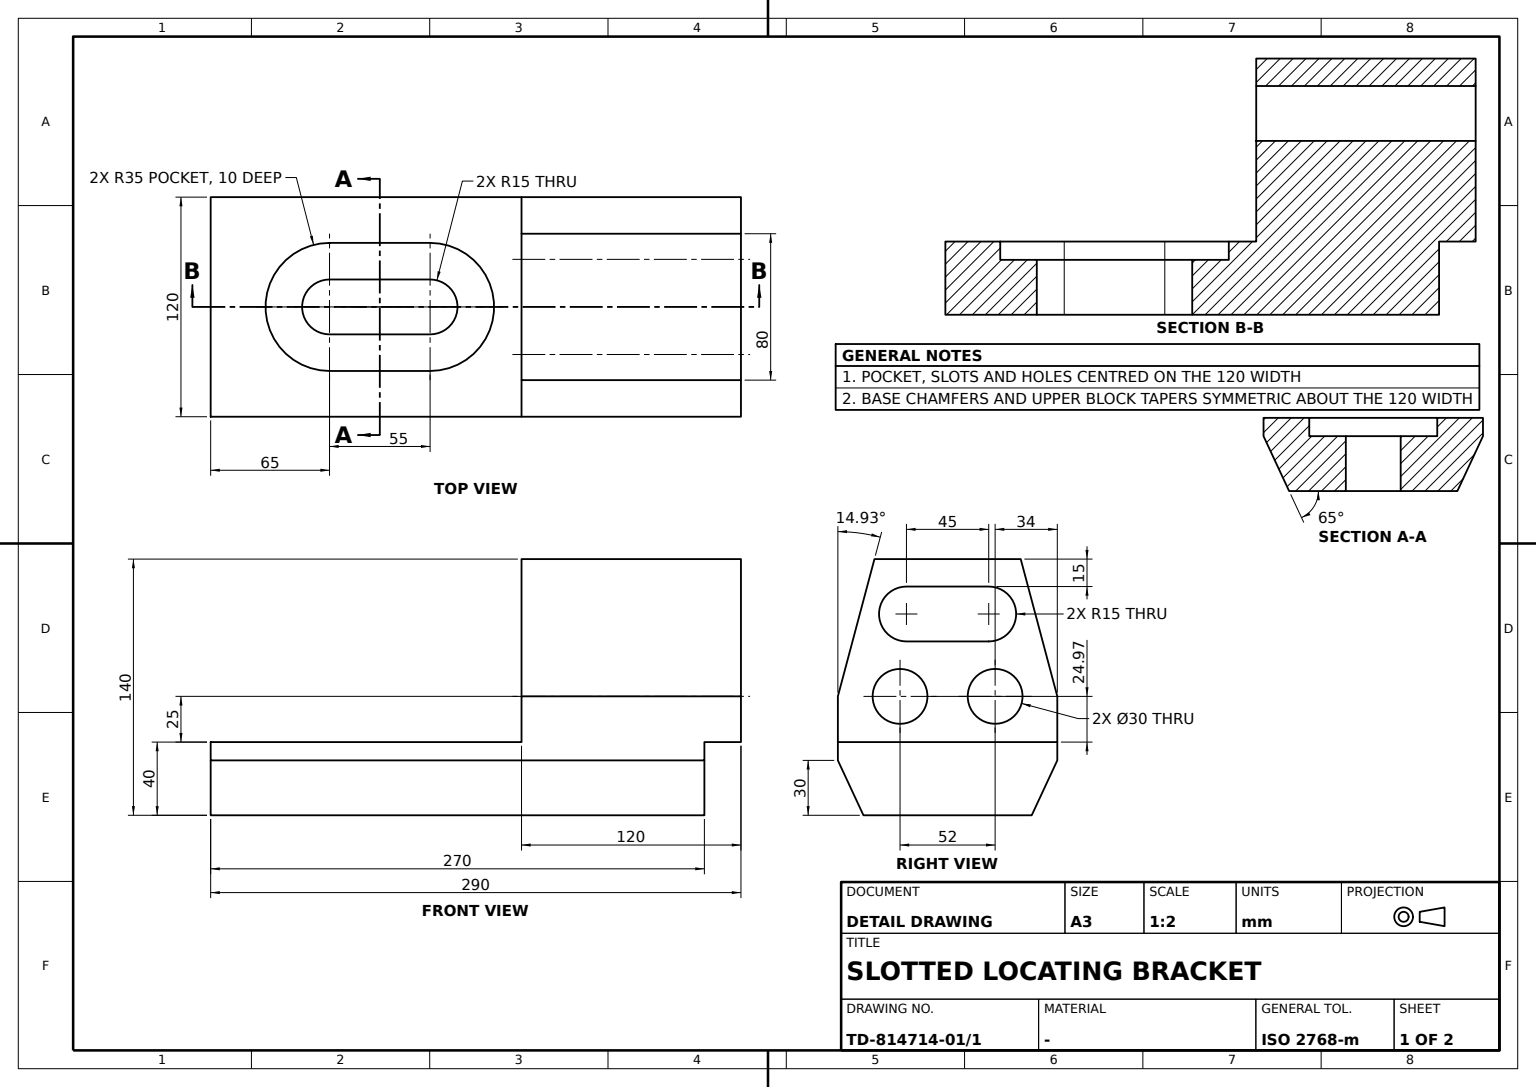
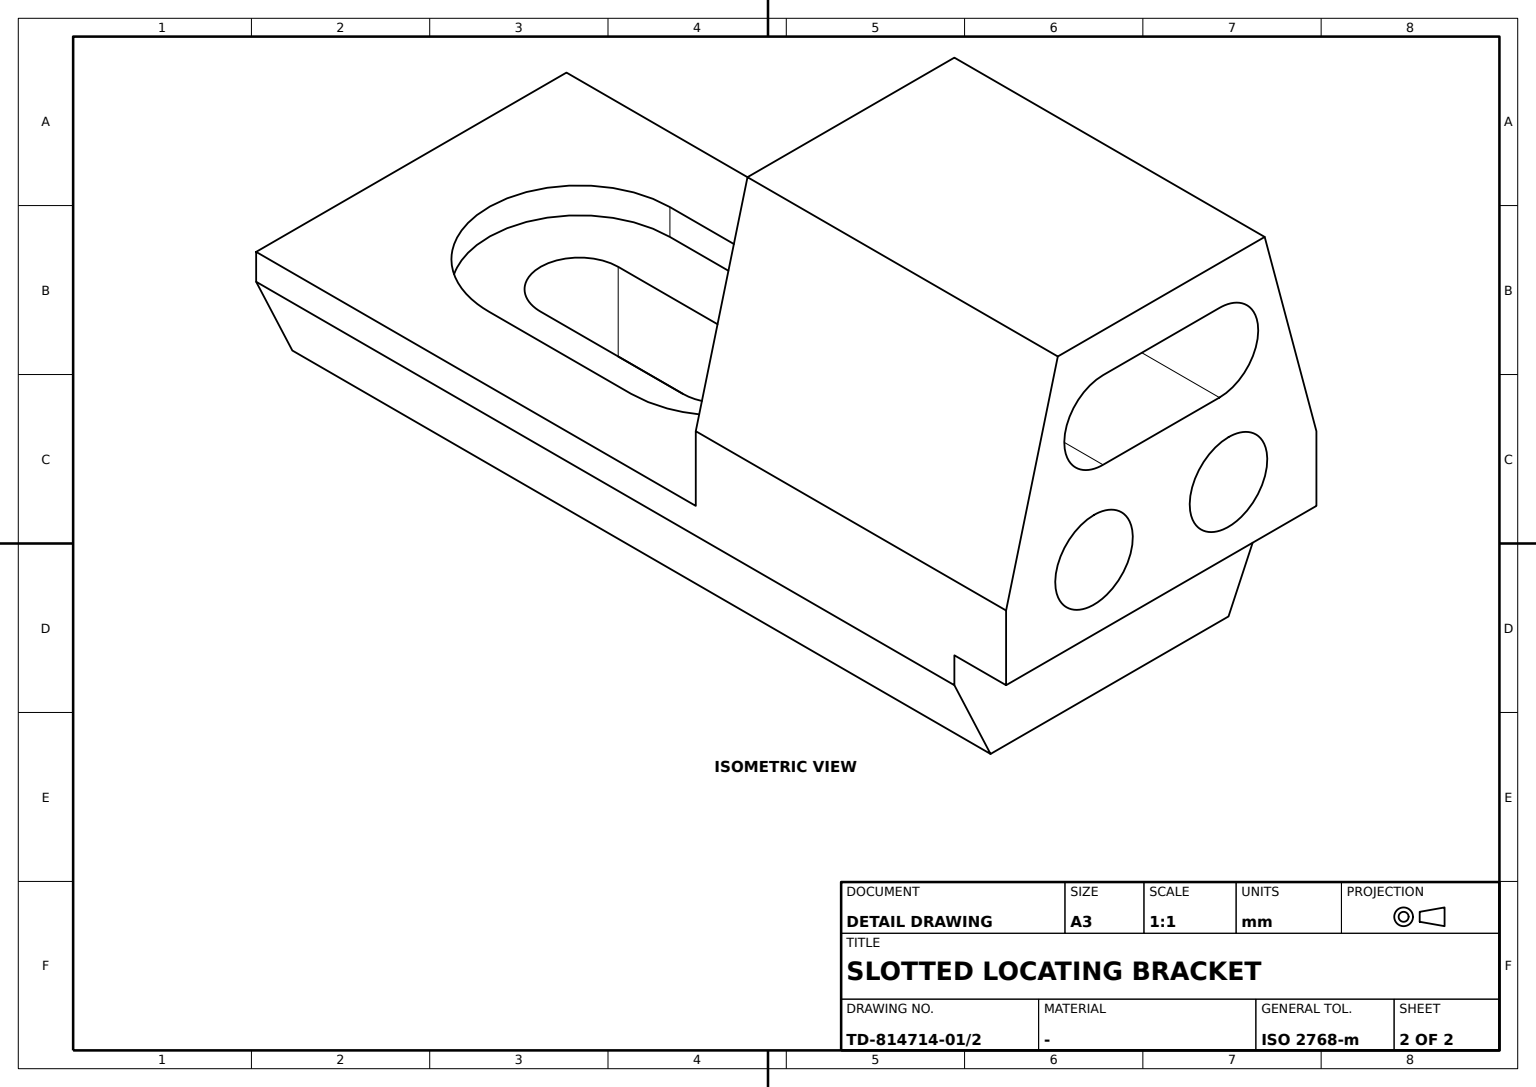
ISO-10303-21;
HEADER;
FILE_DESCRIPTION((''),'2;1');
FILE_NAME('','',(''),(''),'','','');
FILE_SCHEMA(('AUTOMOTIVE_DESIGN'));
ENDSEC;
DATA;
#1=APPLICATION_CONTEXT('');
#2=PRODUCT_CONTEXT('',#1,'mechanical');
#3=PRODUCT('','','',(#2));
#4=PRODUCT_DEFINITION_FORMATION('','',#3);
#5=PRODUCT_DEFINITION_CONTEXT('',#1,'design');
#6=PRODUCT_DEFINITION('','',#4,#5);
#7=PRODUCT_DEFINITION_SHAPE('','',#6);
#8=(LENGTH_UNIT()NAMED_UNIT(*)SI_UNIT(.MILLI.,.METRE.));
#9=(NAMED_UNIT(*)PLANE_ANGLE_UNIT()SI_UNIT($,.RADIAN.));
#10=(NAMED_UNIT(*)SI_UNIT($,.STERADIAN.)SOLID_ANGLE_UNIT());
#11=UNCERTAINTY_MEASURE_WITH_UNIT(LENGTH_MEASURE(0.005),#8,'distance_accuracy_value','');
#12=(GEOMETRIC_REPRESENTATION_CONTEXT(3)GLOBAL_UNCERTAINTY_ASSIGNED_CONTEXT((#11))GLOBAL_UNIT_ASSIGNED_CONTEXT((#8,#9,#10))REPRESENTATION_CONTEXT('',''));
#13=CARTESIAN_POINT('',(26.,155.,79.972917));
#14=VERTEX_POINT('',#13);
#15=CARTESIAN_POINT('',(26.,155.,64.972917));
#16=DIRECTION('',(0.,1.,0.));
#17=DIRECTION('',(0.,0.,1.));
#18=AXIS2_PLACEMENT_3D('',#15,#16,#17);
#19=CIRCLE('',#18,15.);
#20=EDGE_CURVE('',#14,#14,#19,.T.);
#21=ORIENTED_EDGE('',*,*,#20,.T.);
#22=EDGE_LOOP('',(#21));
#23=FACE_BOUND('',#22,.T.);
#24=CARTESIAN_POINT('',(26.,35.,79.972917));
#25=VERTEX_POINT('',#24);
#26=CARTESIAN_POINT('',(26.,35.,64.972917));
#27=AXIS2_PLACEMENT_3D('',#26,#16,#17);
#28=CIRCLE('',#27,15.);
#29=EDGE_CURVE('',#25,#25,#28,.T.);
#30=ORIENTED_EDGE('',*,*,#29,.F.);
#31=EDGE_LOOP('',(#30));
#32=FACE_BOUND('',#31,.T.);
#33=CYLINDRICAL_SURFACE('',#27,15.);
#34=ADVANCED_FACE('',(#23,#32),#33,.F.);
#35=CARTESIAN_POINT('',(-60.,135.,30.));
#36=VERTEX_POINT('',#35);
#37=CARTESIAN_POINT('',(-60.,135.,40.));
#38=VERTEX_POINT('',#37);
#39=VECTOR('',#17,1000.);
#40=LINE('',#35,#39);
#41=EDGE_CURVE('',#36,#38,#40,.T.);
#42=ORIENTED_EDGE('',*,*,#41,.F.);
#43=CARTESIAN_POINT('',(-60.,-135.,30.));
#44=VERTEX_POINT('',#43);
#45=VECTOR('',#16,1000.);
#46=LINE('',#43,#45);
#47=EDGE_CURVE('',#44,#36,#46,.T.);
#48=ORIENTED_EDGE('',*,*,#47,.F.);
#49=CARTESIAN_POINT('',(-60.,-135.,40.));
#50=VERTEX_POINT('',#49);
#51=LINE('',#43,#39);
#52=EDGE_CURVE('',#44,#50,#51,.T.);
#53=ORIENTED_EDGE('',*,*,#52,.T.);
#54=CARTESIAN_POINT('',(-60.,35.,40.));
#55=VERTEX_POINT('',#54);
#56=LINE('',#49,#45);
#57=EDGE_CURVE('',#50,#55,#56,.T.);
#58=ORIENTED_EDGE('',*,*,#57,.T.);
#59=CARTESIAN_POINT('',(-60.,35.,65.));
#60=VERTEX_POINT('',#59);
#61=LINE('',#54,#39);
#62=EDGE_CURVE('',#55,#60,#61,.T.);
#63=ORIENTED_EDGE('',*,*,#62,.T.);
#64=CARTESIAN_POINT('',(-60.,155.,65.));
#65=VERTEX_POINT('',#64);
#66=DIRECTION('',(0.,-1.,0.));
#67=VECTOR('',#66,1000.);
#68=LINE('',#64,#67);
#69=EDGE_CURVE('',#65,#60,#68,.T.);
#70=ORIENTED_EDGE('',*,*,#69,.F.);
#71=CARTESIAN_POINT('',(-60.,155.,40.));
#72=VERTEX_POINT('',#71);
#73=LINE('',#71,#39);
#74=EDGE_CURVE('',#72,#65,#73,.T.);
#75=ORIENTED_EDGE('',*,*,#74,.F.);
#76=LINE('',#71,#67);
#77=EDGE_CURVE('',#72,#38,#76,.T.);
#78=ORIENTED_EDGE('',*,*,#77,.T.);
#79=EDGE_LOOP('',(#42,#48,#53,#58,#63,#70,#75,#78));
#80=FACE_BOUND('',#79,.T.);
#81=DIRECTION('',(-1.,0.,0.));
#82=AXIS2_PLACEMENT_3D('',#43,#81,#17);
#83=PLANE('',#82);
#84=ADVANCED_FACE('',(#80),#83,.T.);
#85=CARTESIAN_POINT('',(-15.,-15.,0.));
#86=VERTEX_POINT('',#85);
#87=CARTESIAN_POINT('',(-15.,-15.,30.));
#88=VERTEX_POINT('',#87);
#89=CARTESIAN_POINT('',(-15.,-15.,65.));
#90=DIRECTION('',(0.,0.,-1.));
#91=VECTOR('',#90,1000.);
#92=LINE('',#89,#91);
#93=EDGE_CURVE('',#86,#88,#92,.F.);
#94=ORIENTED_EDGE('',*,*,#93,.F.);
#95=CARTESIAN_POINT('',(15.,-15.,0.));
#96=VERTEX_POINT('',#95);
#97=CARTESIAN_POINT('',(0.,-15.,0.));
#98=AXIS2_PLACEMENT_3D('',#97,#90,#81);
#99=CIRCLE('',#98,15.);
#100=EDGE_CURVE('',#96,#86,#99,.F.);
#101=ORIENTED_EDGE('',*,*,#100,.F.);
#102=CARTESIAN_POINT('',(15.,-15.,30.));
#103=VERTEX_POINT('',#102);
#104=CARTESIAN_POINT('',(15.,-15.,65.));
#105=LINE('',#104,#91);
#106=EDGE_CURVE('',#96,#103,#105,.F.);
#107=ORIENTED_EDGE('',*,*,#106,.T.);
#108=CARTESIAN_POINT('',(0.,-15.,30.));
#109=DIRECTION('',(1.,0.,0.));
#110=AXIS2_PLACEMENT_3D('',#108,#17,#109);
#111=CIRCLE('',#110,15.);
#112=EDGE_CURVE('',#88,#103,#111,.F.);
#113=ORIENTED_EDGE('',*,*,#112,.F.);
#114=EDGE_LOOP('',(#94,#101,#107,#113));
#115=FACE_BOUND('',#114,.T.);
#116=CARTESIAN_POINT('',(0.,-15.,65.));
#117=AXIS2_PLACEMENT_3D('',#116,#90,#81);
#118=CYLINDRICAL_SURFACE('',#117,15.);
#119=ADVANCED_FACE('',(#115),#118,.F.);
#120=CARTESIAN_POINT('',(46.01077,135.,0.));
#121=VERTEX_POINT('',#120);
#122=CARTESIAN_POINT('',(-46.01077,135.,0.));
#123=VERTEX_POINT('',#122);
#124=VECTOR('',#81,1000.);
#125=LINE('',#120,#124);
#126=EDGE_CURVE('',#121,#123,#125,.T.);
#127=ORIENTED_EDGE('',*,*,#126,.T.);
#128=DIRECTION('',(-0.422618262,0.,0.906307787));
#129=VECTOR('',#128,1000.);
#130=LINE('',#122,#129);
#131=EDGE_CURVE('',#123,#36,#130,.T.);
#132=ORIENTED_EDGE('',*,*,#131,.T.);
#133=ORIENTED_EDGE('',*,*,#41,.T.);
#134=CARTESIAN_POINT('',(60.,135.,40.));
#135=VERTEX_POINT('',#134);
#136=VECTOR('',#109,1000.);
#137=LINE('',#37,#136);
#138=EDGE_CURVE('',#38,#135,#137,.T.);
#139=ORIENTED_EDGE('',*,*,#138,.T.);
#140=CARTESIAN_POINT('',(60.,135.,30.));
#141=VERTEX_POINT('',#140);
#142=LINE('',#134,#91);
#143=EDGE_CURVE('',#135,#141,#142,.T.);
#144=ORIENTED_EDGE('',*,*,#143,.T.);
#145=DIRECTION('',(-0.422618262,0.,-0.906307787));
#146=VECTOR('',#145,1000.);
#147=LINE('',#140,#146);
#148=EDGE_CURVE('',#141,#121,#147,.T.);
#149=ORIENTED_EDGE('',*,*,#148,.T.);
#150=EDGE_LOOP('',(#127,#132,#133,#139,#144,#149));
#151=FACE_BOUND('',#150,.T.);
#152=CARTESIAN_POINT('',(0.,135.,0.));
#153=AXIS2_PLACEMENT_3D('',#152,#16,#17);
#154=PLANE('',#153);
#155=ADVANCED_FACE('',(#151),#154,.T.);
#156=CARTESIAN_POINT('',(-26.,35.,80.));
#157=VERTEX_POINT('',#156);
#158=CARTESIAN_POINT('',(-26.,35.,65.));
#159=AXIS2_PLACEMENT_3D('',#158,#16,#17);
#160=CIRCLE('',#159,15.);
#161=EDGE_CURVE('',#157,#157,#160,.T.);
#162=ORIENTED_EDGE('',*,*,#161,.F.);
#163=EDGE_LOOP('',(#162));
#164=FACE_BOUND('',#163,.T.);
#165=CARTESIAN_POINT('',(-26.,155.,80.));
#166=VERTEX_POINT('',#165);
#167=CARTESIAN_POINT('',(-26.,155.,65.));
#168=AXIS2_PLACEMENT_3D('',#167,#16,#17);
#169=CIRCLE('',#168,15.);
#170=EDGE_CURVE('',#166,#166,#169,.T.);
#171=ORIENTED_EDGE('',*,*,#170,.T.);
#172=EDGE_LOOP('',(#171));
#173=FACE_BOUND('',#172,.T.);
#174=CYLINDRICAL_SURFACE('',#159,15.);
#175=ADVANCED_FACE('',(#164,#173),#174,.F.);
#176=CARTESIAN_POINT('',(15.,-70.,0.));
#177=VERTEX_POINT('',#176);
#178=CARTESIAN_POINT('',(15.,-70.,30.));
#179=VERTEX_POINT('',#178);
#180=CARTESIAN_POINT('',(15.,-70.,65.));
#181=LINE('',#180,#91);
#182=EDGE_CURVE('',#177,#179,#181,.F.);
#183=ORIENTED_EDGE('',*,*,#182,.T.);
#184=LINE('',#178,#67);
#185=EDGE_CURVE('',#103,#179,#184,.T.);
#186=ORIENTED_EDGE('',*,*,#185,.F.);
#187=ORIENTED_EDGE('',*,*,#106,.F.);
#188=CARTESIAN_POINT('',(15.,-135.,0.));
#189=LINE('',#188,#45);
#190=EDGE_CURVE('',#177,#96,#189,.T.);
#191=ORIENTED_EDGE('',*,*,#190,.F.);
#192=EDGE_LOOP('',(#183,#186,#187,#191));
#193=FACE_BOUND('',#192,.T.);
#194=AXIS2_PLACEMENT_3D('',#180,#81,#66);
#195=PLANE('',#194);
#196=ADVANCED_FACE('',(#193),#195,.T.);
#197=CARTESIAN_POINT('',(22.5,35.,95.));
#198=VERTEX_POINT('',#197);
#199=CARTESIAN_POINT('',(22.5,155.,95.));
#200=VERTEX_POINT('',#199);
#201=CARTESIAN_POINT('',(22.5,212.,95.));
#202=LINE('',#201,#67);
#203=EDGE_CURVE('',#198,#200,#202,.F.);
#204=ORIENTED_EDGE('',*,*,#203,.F.);
#205=CARTESIAN_POINT('',(22.5,35.,125.));
#206=VERTEX_POINT('',#205);
#207=CARTESIAN_POINT('',(22.5,35.,110.));
#208=AXIS2_PLACEMENT_3D('',#207,#16,#17);
#209=CIRCLE('',#208,15.);
#210=EDGE_CURVE('',#206,#198,#209,.T.);
#211=ORIENTED_EDGE('',*,*,#210,.F.);
#212=CARTESIAN_POINT('',(22.5,155.,125.));
#213=VERTEX_POINT('',#212);
#214=CARTESIAN_POINT('',(22.5,212.,125.));
#215=LINE('',#214,#67);
#216=EDGE_CURVE('',#206,#213,#215,.F.);
#217=ORIENTED_EDGE('',*,*,#216,.T.);
#218=CARTESIAN_POINT('',(22.5,155.,110.));
#219=AXIS2_PLACEMENT_3D('',#218,#16,#17);
#220=CIRCLE('',#219,15.);
#221=EDGE_CURVE('',#213,#200,#220,.T.);
#222=ORIENTED_EDGE('',*,*,#221,.T.);
#223=EDGE_LOOP('',(#204,#211,#217,#222));
#224=FACE_BOUND('',#223,.T.);
#225=CARTESIAN_POINT('',(22.5,212.,110.));
#226=AXIS2_PLACEMENT_3D('',#225,#66,#90);
#227=CYLINDRICAL_SURFACE('',#226,15.);
#228=ADVANCED_FACE('',(#224),#227,.F.);
#229=CARTESIAN_POINT('',(-40.,155.,140.));
#230=VERTEX_POINT('',#229);
#231=CARTESIAN_POINT('',(-40.,35.,140.));
#232=VERTEX_POINT('',#231);
#233=LINE('',#229,#67);
#234=EDGE_CURVE('',#230,#232,#233,.T.);
#235=ORIENTED_EDGE('',*,*,#234,.T.);
#236=CARTESIAN_POINT('',(40.,35.,140.));
#237=VERTEX_POINT('',#236);
#238=LINE('',#231,#136);
#239=EDGE_CURVE('',#232,#237,#238,.T.);
#240=ORIENTED_EDGE('',*,*,#239,.T.);
#241=CARTESIAN_POINT('',(40.,155.,140.));
#242=VERTEX_POINT('',#241);
#243=LINE('',#241,#67);
#244=EDGE_CURVE('',#242,#237,#243,.T.);
#245=ORIENTED_EDGE('',*,*,#244,.F.);
#246=LINE('',#229,#136);
#247=EDGE_CURVE('',#230,#242,#246,.T.);
#248=ORIENTED_EDGE('',*,*,#247,.F.);
#249=EDGE_LOOP('',(#235,#240,#245,#248));
#250=FACE_BOUND('',#249,.T.);
#251=AXIS2_PLACEMENT_3D('',#229,#90,#81);
#252=PLANE('',#251);
#253=ADVANCED_FACE('',(#250),#252,.F.);
#254=CARTESIAN_POINT('',(-35.,-15.,30.));
#255=VERTEX_POINT('',#254);
#256=CARTESIAN_POINT('',(35.,-15.,30.));
#257=VERTEX_POINT('',#256);
#258=CIRCLE('',#110,35.);
#259=EDGE_CURVE('',#255,#257,#258,.F.);
#260=ORIENTED_EDGE('',*,*,#259,.F.);
#261=CARTESIAN_POINT('',(-35.,-70.,30.));
#262=VERTEX_POINT('',#261);
#263=LINE('',#254,#67);
#264=EDGE_CURVE('',#262,#255,#263,.F.);
#265=ORIENTED_EDGE('',*,*,#264,.F.);
#266=CARTESIAN_POINT('',(35.,-70.,30.));
#267=VERTEX_POINT('',#266);
#268=CARTESIAN_POINT('',(0.,-70.,30.));
#269=AXIS2_PLACEMENT_3D('',#268,#17,#109);
#270=CIRCLE('',#269,35.);
#271=EDGE_CURVE('',#267,#262,#270,.F.);
#272=ORIENTED_EDGE('',*,*,#271,.F.);
#273=LINE('',#266,#45);
#274=EDGE_CURVE('',#257,#267,#273,.F.);
#275=ORIENTED_EDGE('',*,*,#274,.F.);
#276=EDGE_LOOP('',(#260,#265,#272,#275));
#277=FACE_BOUND('',#276,.T.);
#278=CARTESIAN_POINT('',(-15.,-70.,30.));
#279=VERTEX_POINT('',#278);
#280=LINE('',#278,#45);
#281=EDGE_CURVE('',#279,#88,#280,.T.);
#282=ORIENTED_EDGE('',*,*,#281,.T.);
#283=ORIENTED_EDGE('',*,*,#112,.T.);
#284=ORIENTED_EDGE('',*,*,#185,.T.);
#285=CIRCLE('',#269,15.);
#286=EDGE_CURVE('',#179,#279,#285,.F.);
#287=ORIENTED_EDGE('',*,*,#286,.T.);
#288=EDGE_LOOP('',(#282,#283,#284,#287));
#289=FACE_BOUND('',#288,.T.);
#290=PLANE('',#269);
#291=ADVANCED_FACE('',(#277,#289),#290,.T.);
#292=CARTESIAN_POINT('',(35.,-15.,40.));
#293=VERTEX_POINT('',#292);
#294=CARTESIAN_POINT('',(35.,-70.,40.));
#295=VERTEX_POINT('',#294);
#296=CARTESIAN_POINT('',(35.,-135.,40.));
#297=LINE('',#296,#67);
#298=EDGE_CURVE('',#293,#295,#297,.T.);
#299=ORIENTED_EDGE('',*,*,#298,.T.);
#300=CARTESIAN_POINT('',(-35.,-70.,40.));
#301=VERTEX_POINT('',#300);
#302=CARTESIAN_POINT('',(0.,-70.,40.));
#303=AXIS2_PLACEMENT_3D('',#302,#17,#109);
#304=CIRCLE('',#303,35.);
#305=EDGE_CURVE('',#295,#301,#304,.F.);
#306=ORIENTED_EDGE('',*,*,#305,.T.);
#307=CARTESIAN_POINT('',(-35.,-15.,40.));
#308=VERTEX_POINT('',#307);
#309=CARTESIAN_POINT('',(-35.,-135.,40.));
#310=LINE('',#309,#45);
#311=EDGE_CURVE('',#301,#308,#310,.T.);
#312=ORIENTED_EDGE('',*,*,#311,.T.);
#313=CARTESIAN_POINT('',(0.,-15.,40.));
#314=AXIS2_PLACEMENT_3D('',#313,#17,#109);
#315=CIRCLE('',#314,35.);
#316=EDGE_CURVE('',#308,#293,#315,.F.);
#317=ORIENTED_EDGE('',*,*,#316,.T.);
#318=EDGE_LOOP('',(#299,#306,#312,#317));
#319=FACE_BOUND('',#318,.T.);
#320=CARTESIAN_POINT('',(60.,35.,40.));
#321=VERTEX_POINT('',#320);
#322=LINE('',#320,#124);
#323=EDGE_CURVE('',#321,#55,#322,.T.);
#324=ORIENTED_EDGE('',*,*,#323,.T.);
#325=ORIENTED_EDGE('',*,*,#57,.F.);
#326=CARTESIAN_POINT('',(60.,-135.,40.));
#327=VERTEX_POINT('',#326);
#328=LINE('',#49,#136);
#329=EDGE_CURVE('',#50,#327,#328,.T.);
#330=ORIENTED_EDGE('',*,*,#329,.T.);
#331=LINE('',#326,#45);
#332=EDGE_CURVE('',#327,#321,#331,.T.);
#333=ORIENTED_EDGE('',*,*,#332,.T.);
#334=EDGE_LOOP('',(#324,#325,#330,#333));
#335=FACE_BOUND('',#334,.T.);
#336=AXIS2_PLACEMENT_3D('',#49,#17,#109);
#337=PLANE('',#336);
#338=ADVANCED_FACE('',(#319,#335),#337,.T.);
#339=ORIENTED_EDGE('',*,*,#239,.F.);
#340=DIRECTION('',(0.257662651,0.,0.96623494));
#341=VECTOR('',#340,1000.);
#342=LINE('',#59,#341);
#343=EDGE_CURVE('',#60,#232,#342,.T.);
#344=ORIENTED_EDGE('',*,*,#343,.F.);
#345=ORIENTED_EDGE('',*,*,#62,.F.);
#346=ORIENTED_EDGE('',*,*,#323,.F.);
#347=CARTESIAN_POINT('',(60.,35.,65.));
#348=VERTEX_POINT('',#347);
#349=LINE('',#347,#91);
#350=EDGE_CURVE('',#348,#321,#349,.T.);
#351=ORIENTED_EDGE('',*,*,#350,.F.);
#352=DIRECTION('',(0.257662651,0.,-0.96623494));
#353=VECTOR('',#352,1000.);
#354=LINE('',#236,#353);
#355=EDGE_CURVE('',#237,#348,#354,.T.);
#356=ORIENTED_EDGE('',*,*,#355,.F.);
#357=EDGE_LOOP('',(#339,#344,#345,#346,#351,#356));
#358=FACE_BOUND('',#357,.T.);
#359=ORIENTED_EDGE('',*,*,#29,.T.);
#360=EDGE_LOOP('',(#359));
#361=FACE_BOUND('',#360,.T.);
#362=CARTESIAN_POINT('',(-22.5,35.,125.));
#363=VERTEX_POINT('',#362);
#364=CARTESIAN_POINT('',(0.,35.,125.));
#365=LINE('',#364,#136);
#366=EDGE_CURVE('',#363,#206,#365,.T.);
#367=ORIENTED_EDGE('',*,*,#366,.T.);
#368=ORIENTED_EDGE('',*,*,#210,.T.);
#369=CARTESIAN_POINT('',(-22.5,35.,95.));
#370=VERTEX_POINT('',#369);
#371=CARTESIAN_POINT('',(0.,35.,95.));
#372=LINE('',#371,#124);
#373=EDGE_CURVE('',#198,#370,#372,.T.);
#374=ORIENTED_EDGE('',*,*,#373,.T.);
#375=CARTESIAN_POINT('',(-22.5,35.,110.));
#376=AXIS2_PLACEMENT_3D('',#375,#16,#17);
#377=CIRCLE('',#376,15.);
#378=EDGE_CURVE('',#370,#363,#377,.T.);
#379=ORIENTED_EDGE('',*,*,#378,.T.);
#380=EDGE_LOOP('',(#367,#368,#374,#379));
#381=FACE_BOUND('',#380,.T.);
#382=ORIENTED_EDGE('',*,*,#161,.T.);
#383=EDGE_LOOP('',(#382));
#384=FACE_BOUND('',#383,.T.);
#385=CARTESIAN_POINT('',(0.,35.,0.));
#386=AXIS2_PLACEMENT_3D('',#385,#16,#17);
#387=PLANE('',#386);
#388=ADVANCED_FACE('',(#358,#361,#381,#384),#387,.F.);
#389=CARTESIAN_POINT('',(60.,155.,40.));
#390=VERTEX_POINT('',#389);
#391=LINE('',#389,#67);
#392=EDGE_CURVE('',#390,#135,#391,.T.);
#393=ORIENTED_EDGE('',*,*,#392,.T.);
#394=ORIENTED_EDGE('',*,*,#138,.F.);
#395=ORIENTED_EDGE('',*,*,#77,.F.);
#396=LINE('',#389,#124);
#397=EDGE_CURVE('',#390,#72,#396,.T.);
#398=ORIENTED_EDGE('',*,*,#397,.F.);
#399=EDGE_LOOP('',(#393,#394,#395,#398));
#400=FACE_BOUND('',#399,.T.);
#401=AXIS2_PLACEMENT_3D('',#389,#17,#109);
#402=PLANE('',#401);
#403=ADVANCED_FACE('',(#400),#402,.F.);
#404=ORIENTED_EDGE('',*,*,#264,.T.);
#405=CARTESIAN_POINT('',(-35.,-15.,65.));
#406=LINE('',#405,#91);
#407=EDGE_CURVE('',#255,#308,#406,.F.);
#408=ORIENTED_EDGE('',*,*,#407,.T.);
#409=ORIENTED_EDGE('',*,*,#311,.F.);
#410=CARTESIAN_POINT('',(-35.,-70.,65.));
#411=LINE('',#410,#91);
#412=EDGE_CURVE('',#262,#301,#411,.F.);
#413=ORIENTED_EDGE('',*,*,#412,.F.);
#414=EDGE_LOOP('',(#404,#408,#409,#413));
#415=FACE_BOUND('',#414,.T.);
#416=AXIS2_PLACEMENT_3D('',#405,#109,#16);
#417=PLANE('',#416);
#418=ADVANCED_FACE('',(#415),#417,.T.);
#419=CARTESIAN_POINT('',(-46.01077,-135.,0.));
#420=VERTEX_POINT('',#419);
#421=LINE('',#419,#45);
#422=EDGE_CURVE('',#420,#123,#421,.T.);
#423=ORIENTED_EDGE('',*,*,#422,.F.);
#424=LINE('',#419,#129);
#425=EDGE_CURVE('',#420,#44,#424,.T.);
#426=ORIENTED_EDGE('',*,*,#425,.T.);
#427=ORIENTED_EDGE('',*,*,#47,.T.);
#428=ORIENTED_EDGE('',*,*,#131,.F.);
#429=EDGE_LOOP('',(#423,#426,#427,#428));
#430=FACE_BOUND('',#429,.T.);
#431=DIRECTION('',(-0.906307787,0.,-0.422618262));
#432=AXIS2_PLACEMENT_3D('',#419,#431,#128);
#433=PLANE('',#432);
#434=ADVANCED_FACE('',(#430),#433,.T.);
#435=ORIENTED_EDGE('',*,*,#425,.F.);
#436=CARTESIAN_POINT('',(46.01077,-135.,0.));
#437=VERTEX_POINT('',#436);
#438=LINE('',#436,#124);
#439=EDGE_CURVE('',#437,#420,#438,.T.);
#440=ORIENTED_EDGE('',*,*,#439,.F.);
#441=CARTESIAN_POINT('',(60.,-135.,30.));
#442=VERTEX_POINT('',#441);
#443=LINE('',#441,#146);
#444=EDGE_CURVE('',#442,#437,#443,.T.);
#445=ORIENTED_EDGE('',*,*,#444,.F.);
#446=LINE('',#326,#91);
#447=EDGE_CURVE('',#327,#442,#446,.T.);
#448=ORIENTED_EDGE('',*,*,#447,.F.);
#449=ORIENTED_EDGE('',*,*,#329,.F.);
#450=ORIENTED_EDGE('',*,*,#52,.F.);
#451=EDGE_LOOP('',(#435,#440,#445,#448,#449,#450));
#452=FACE_BOUND('',#451,.T.);
#453=CARTESIAN_POINT('',(0.,-135.,0.));
#454=AXIS2_PLACEMENT_3D('',#453,#16,#17);
#455=PLANE('',#454);
#456=ADVANCED_FACE('',(#452),#455,.F.);
#457=ORIENTED_EDGE('',*,*,#93,.T.);
#458=ORIENTED_EDGE('',*,*,#281,.F.);
#459=CARTESIAN_POINT('',(-15.,-70.,0.));
#460=VERTEX_POINT('',#459);
#461=CARTESIAN_POINT('',(-15.,-70.,65.));
#462=LINE('',#461,#91);
#463=EDGE_CURVE('',#460,#279,#462,.F.);
#464=ORIENTED_EDGE('',*,*,#463,.F.);
#465=CARTESIAN_POINT('',(-15.,-135.,0.));
#466=LINE('',#465,#67);
#467=EDGE_CURVE('',#86,#460,#466,.T.);
#468=ORIENTED_EDGE('',*,*,#467,.F.);
#469=EDGE_LOOP('',(#457,#458,#464,#468));
#470=FACE_BOUND('',#469,.T.);
#471=AXIS2_PLACEMENT_3D('',#89,#109,#16);
#472=PLANE('',#471);
#473=ADVANCED_FACE('',(#470),#472,.T.);
#474=ORIENTED_EDGE('',*,*,#343,.T.);
#475=ORIENTED_EDGE('',*,*,#234,.F.);
#476=LINE('',#64,#341);
#477=EDGE_CURVE('',#65,#230,#476,.T.);
#478=ORIENTED_EDGE('',*,*,#477,.F.);
#479=ORIENTED_EDGE('',*,*,#69,.T.);
#480=EDGE_LOOP('',(#474,#475,#478,#479));
#481=FACE_BOUND('',#480,.T.);
#482=DIRECTION('',(0.96623494,0.,-0.257662651));
#483=DIRECTION('',(-0.257662651,0.,-0.96623494));
#484=AXIS2_PLACEMENT_3D('',#64,#482,#483);
#485=PLANE('',#484);
#486=ADVANCED_FACE('',(#481),#485,.F.);
#487=ORIENTED_EDGE('',*,*,#463,.T.);
#488=ORIENTED_EDGE('',*,*,#286,.F.);
#489=ORIENTED_EDGE('',*,*,#182,.F.);
#490=CARTESIAN_POINT('',(0.,-70.,0.));
#491=AXIS2_PLACEMENT_3D('',#490,#90,#81);
#492=CIRCLE('',#491,15.);
#493=EDGE_CURVE('',#460,#177,#492,.F.);
#494=ORIENTED_EDGE('',*,*,#493,.F.);
#495=EDGE_LOOP('',(#487,#488,#489,#494));
#496=FACE_BOUND('',#495,.T.);
#497=CARTESIAN_POINT('',(0.,-70.,65.));
#498=AXIS2_PLACEMENT_3D('',#497,#90,#81);
#499=CYLINDRICAL_SURFACE('',#498,15.);
#500=ADVANCED_FACE('',(#496),#499,.F.);
#501=ORIENTED_EDGE('',*,*,#439,.T.);
#502=ORIENTED_EDGE('',*,*,#422,.T.);
#503=ORIENTED_EDGE('',*,*,#126,.F.);
#504=LINE('',#436,#45);
#505=EDGE_CURVE('',#437,#121,#504,.T.);
#506=ORIENTED_EDGE('',*,*,#505,.F.);
#507=EDGE_LOOP('',(#501,#502,#503,#506));
#508=FACE_BOUND('',#507,.T.);
#509=ORIENTED_EDGE('',*,*,#493,.T.);
#510=ORIENTED_EDGE('',*,*,#190,.T.);
#511=ORIENTED_EDGE('',*,*,#100,.T.);
#512=ORIENTED_EDGE('',*,*,#467,.T.);
#513=EDGE_LOOP('',(#509,#510,#511,#512));
#514=FACE_BOUND('',#513,.T.);
#515=AXIS2_PLACEMENT_3D('',#436,#90,#81);
#516=PLANE('',#515);
#517=ADVANCED_FACE('',(#508,#514),#516,.T.);
#518=CARTESIAN_POINT('',(35.,-70.,65.));
#519=LINE('',#518,#91);
#520=EDGE_CURVE('',#267,#295,#519,.F.);
#521=ORIENTED_EDGE('',*,*,#520,.F.);
#522=ORIENTED_EDGE('',*,*,#271,.T.);
#523=ORIENTED_EDGE('',*,*,#412,.T.);
#524=ORIENTED_EDGE('',*,*,#305,.F.);
#525=EDGE_LOOP('',(#521,#522,#523,#524));
#526=FACE_BOUND('',#525,.T.);
#527=CYLINDRICAL_SURFACE('',#498,35.);
#528=ADVANCED_FACE('',(#526),#527,.F.);
#529=ORIENTED_EDGE('',*,*,#350,.T.);
#530=ORIENTED_EDGE('',*,*,#332,.F.);
#531=ORIENTED_EDGE('',*,*,#447,.T.);
#532=LINE('',#441,#45);
#533=EDGE_CURVE('',#442,#141,#532,.T.);
#534=ORIENTED_EDGE('',*,*,#533,.T.);
#535=ORIENTED_EDGE('',*,*,#143,.F.);
#536=ORIENTED_EDGE('',*,*,#392,.F.);
#537=CARTESIAN_POINT('',(60.,155.,65.));
#538=VERTEX_POINT('',#537);
#539=LINE('',#537,#91);
#540=EDGE_CURVE('',#538,#390,#539,.T.);
#541=ORIENTED_EDGE('',*,*,#540,.F.);
#542=LINE('',#537,#67);
#543=EDGE_CURVE('',#538,#348,#542,.T.);
#544=ORIENTED_EDGE('',*,*,#543,.T.);
#545=EDGE_LOOP('',(#529,#530,#531,#534,#535,#536,#541,#544));
#546=FACE_BOUND('',#545,.T.);
#547=AXIS2_PLACEMENT_3D('',#326,#109,#90);
#548=PLANE('',#547);
#549=ADVANCED_FACE('',(#546),#548,.T.);
#550=LINE('',#241,#353);
#551=EDGE_CURVE('',#242,#538,#550,.T.);
#552=ORIENTED_EDGE('',*,*,#551,.F.);
#553=ORIENTED_EDGE('',*,*,#244,.T.);
#554=ORIENTED_EDGE('',*,*,#355,.T.);
#555=ORIENTED_EDGE('',*,*,#543,.F.);
#556=EDGE_LOOP('',(#552,#553,#554,#555));
#557=FACE_BOUND('',#556,.T.);
#558=DIRECTION('',(-0.96623494,0.,-0.257662651));
#559=DIRECTION('',(-0.257662651,0.,0.96623494));
#560=AXIS2_PLACEMENT_3D('',#241,#558,#559);
#561=PLANE('',#560);
#562=ADVANCED_FACE('',(#557),#561,.F.);
#563=ORIENTED_EDGE('',*,*,#216,.F.);
#564=ORIENTED_EDGE('',*,*,#366,.F.);
#565=CARTESIAN_POINT('',(-22.5,155.,125.));
#566=VERTEX_POINT('',#565);
#567=CARTESIAN_POINT('',(-22.5,212.,125.));
#568=LINE('',#567,#67);
#569=EDGE_CURVE('',#363,#566,#568,.F.);
#570=ORIENTED_EDGE('',*,*,#569,.T.);
#571=CARTESIAN_POINT('',(0.,155.,125.));
#572=LINE('',#571,#136);
#573=EDGE_CURVE('',#566,#213,#572,.T.);
#574=ORIENTED_EDGE('',*,*,#573,.T.);
#575=EDGE_LOOP('',(#563,#564,#570,#574));
#576=FACE_BOUND('',#575,.T.);
#577=AXIS2_PLACEMENT_3D('',#214,#17,#109);
#578=PLANE('',#577);
#579=ADVANCED_FACE('',(#576),#578,.F.);
#580=ORIENTED_EDGE('',*,*,#520,.T.);
#581=ORIENTED_EDGE('',*,*,#298,.F.);
#582=CARTESIAN_POINT('',(35.,-15.,65.));
#583=LINE('',#582,#91);
#584=EDGE_CURVE('',#257,#293,#583,.F.);
#585=ORIENTED_EDGE('',*,*,#584,.F.);
#586=ORIENTED_EDGE('',*,*,#274,.T.);
#587=EDGE_LOOP('',(#580,#581,#585,#586));
#588=FACE_BOUND('',#587,.T.);
#589=AXIS2_PLACEMENT_3D('',#518,#81,#66);
#590=PLANE('',#589);
#591=ADVANCED_FACE('',(#588),#590,.T.);
#592=ORIENTED_EDGE('',*,*,#584,.T.);
#593=ORIENTED_EDGE('',*,*,#316,.F.);
#594=ORIENTED_EDGE('',*,*,#407,.F.);
#595=ORIENTED_EDGE('',*,*,#259,.T.);
#596=EDGE_LOOP('',(#592,#593,#594,#595));
#597=FACE_BOUND('',#596,.T.);
#598=CYLINDRICAL_SURFACE('',#117,35.);
#599=ADVANCED_FACE('',(#597),#598,.F.);
#600=ORIENTED_EDGE('',*,*,#378,.F.);
#601=CARTESIAN_POINT('',(-22.5,155.,95.));
#602=VERTEX_POINT('',#601);
#603=CARTESIAN_POINT('',(-22.5,212.,95.));
#604=LINE('',#603,#67);
#605=EDGE_CURVE('',#370,#602,#604,.F.);
#606=ORIENTED_EDGE('',*,*,#605,.T.);
#607=CARTESIAN_POINT('',(-22.5,155.,110.));
#608=AXIS2_PLACEMENT_3D('',#607,#16,#17);
#609=CIRCLE('',#608,15.);
#610=EDGE_CURVE('',#602,#566,#609,.T.);
#611=ORIENTED_EDGE('',*,*,#610,.T.);
#612=ORIENTED_EDGE('',*,*,#569,.F.);
#613=EDGE_LOOP('',(#600,#606,#611,#612));
#614=FACE_BOUND('',#613,.T.);
#615=CARTESIAN_POINT('',(-22.5,212.,110.));
#616=AXIS2_PLACEMENT_3D('',#615,#66,#90);
#617=CYLINDRICAL_SURFACE('',#616,15.);
#618=ADVANCED_FACE('',(#614),#617,.F.);
#619=ORIENTED_EDGE('',*,*,#477,.T.);
#620=ORIENTED_EDGE('',*,*,#247,.T.);
#621=ORIENTED_EDGE('',*,*,#551,.T.);
#622=ORIENTED_EDGE('',*,*,#540,.T.);
#623=ORIENTED_EDGE('',*,*,#397,.T.);
#624=ORIENTED_EDGE('',*,*,#74,.T.);
#625=EDGE_LOOP('',(#619,#620,#621,#622,#623,#624));
#626=FACE_BOUND('',#625,.T.);
#627=ORIENTED_EDGE('',*,*,#170,.F.);
#628=EDGE_LOOP('',(#627));
#629=FACE_BOUND('',#628,.T.);
#630=ORIENTED_EDGE('',*,*,#221,.F.);
#631=ORIENTED_EDGE('',*,*,#573,.F.);
#632=ORIENTED_EDGE('',*,*,#610,.F.);
#633=CARTESIAN_POINT('',(0.,155.,95.));
#634=LINE('',#633,#124);
#635=EDGE_CURVE('',#200,#602,#634,.T.);
#636=ORIENTED_EDGE('',*,*,#635,.F.);
#637=EDGE_LOOP('',(#630,#631,#632,#636));
#638=FACE_BOUND('',#637,.T.);
#639=ORIENTED_EDGE('',*,*,#20,.F.);
#640=EDGE_LOOP('',(#639));
#641=FACE_BOUND('',#640,.T.);
#642=CARTESIAN_POINT('',(0.,155.,0.));
#643=AXIS2_PLACEMENT_3D('',#642,#16,#17);
#644=PLANE('',#643);
#645=ADVANCED_FACE('',(#626,#629,#638,#641),#644,.T.);
#646=ORIENTED_EDGE('',*,*,#373,.F.);
#647=ORIENTED_EDGE('',*,*,#203,.T.);
#648=ORIENTED_EDGE('',*,*,#635,.T.);
#649=ORIENTED_EDGE('',*,*,#605,.F.);
#650=EDGE_LOOP('',(#646,#647,#648,#649));
#651=FACE_BOUND('',#650,.T.);
#652=AXIS2_PLACEMENT_3D('',#603,#90,#81);
#653=PLANE('',#652);
#654=ADVANCED_FACE('',(#651),#653,.F.);
#655=ORIENTED_EDGE('',*,*,#533,.F.);
#656=ORIENTED_EDGE('',*,*,#444,.T.);
#657=ORIENTED_EDGE('',*,*,#505,.T.);
#658=ORIENTED_EDGE('',*,*,#148,.F.);
#659=EDGE_LOOP('',(#655,#656,#657,#658));
#660=FACE_BOUND('',#659,.T.);
#661=DIRECTION('',(0.906307787,0.,-0.422618262));
#662=AXIS2_PLACEMENT_3D('',#441,#661,#145);
#663=PLANE('',#662);
#664=ADVANCED_FACE('',(#660),#663,.T.);
#665=CLOSED_SHELL('',(#34,#84,#119,#155,#175,#196,#228,#253,#291,#338,#388,#403,#418,#434,#456,#473,#486,#500,#517,#528,#549,#562,#579,#591,#599,#618,#645,#654,#664));
#666=MANIFOLD_SOLID_BREP('',#665);
#667=ADVANCED_BREP_SHAPE_REPRESENTATION('',(#666),#12);
#668=SHAPE_DEFINITION_REPRESENTATION(#7,#667);
ENDSEC;
END-ISO-10303-21;
